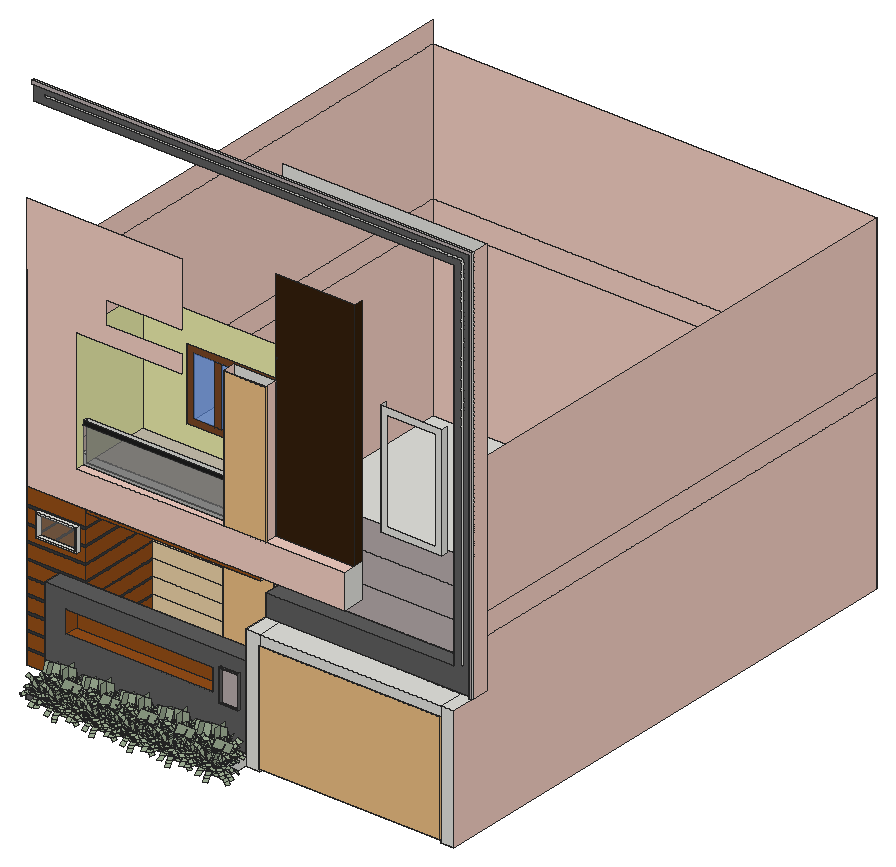
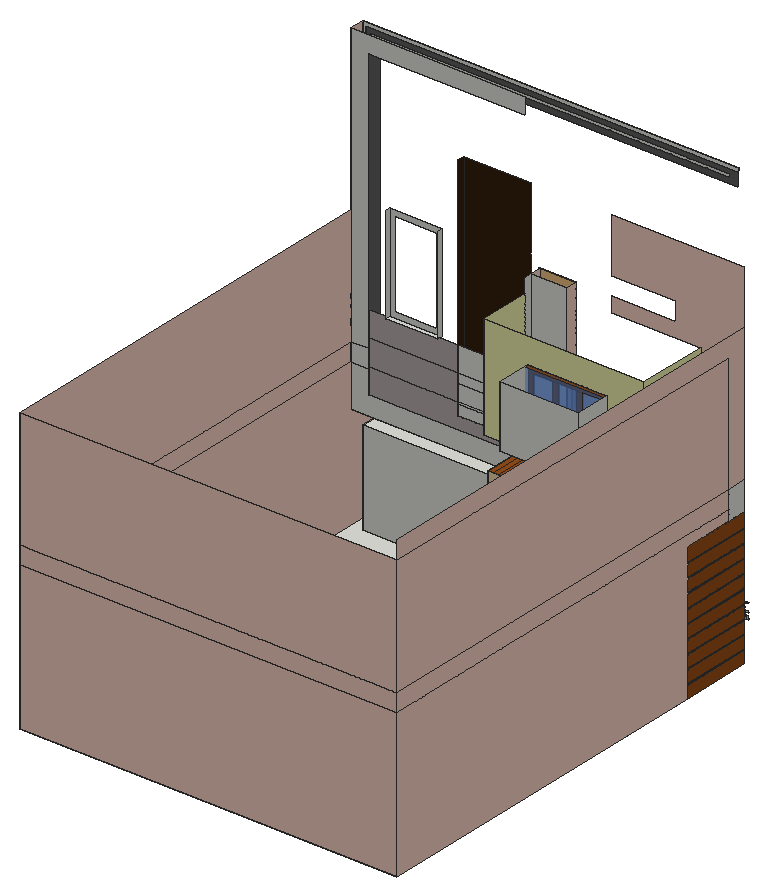
# SketchUp Ruby script. Lengths in inches.
U = 1.inch
M = Sketchup.active_model
def pt(a) = Geom::Point3d.new(a.map { |v| v * U })
def face(e, loops, mat)
  f = e.add_face(loops[0].map { |a| pt(a) })
  loops[1..].each { |l| e.add_face(l.map { |a| pt(a) }).erase! }
  f.material = f.back_material = mat if mat
  f
end
# faces: each face lists its corners as indices into pts; further lists are holes
def faces(e, pts, list, mat = nil) = list.each { |f| face(e, (f[0].is_a?(Array) ? f : [f]).map { |l| l.map { |i| pts[i] } }, mat) }
# xy, xz, yz: faces in a plane at the given z, y or x. An outline is a flat list of corners, or four numbers for a rectangle; further outlines are holes
def ring(l) = l.size == 4 ? [[l[0], l[1]], [l[2], l[1]], [l[2], l[3]], [l[0], l[3]]] : l.each_slice(2).to_a
def flat(e, list, mat, &to3) = list.each { |f| face(e, (f[0].is_a?(Array) ? f : [f]).map { |l| ring(l).map { |u, v| to3.(u, v) } }, mat) }
def xy(e, z, list, mat = nil) = flat(e, list, mat) { |x, y| [x, y, z] }
def xz(e, y, list, mat = nil) = flat(e, list, mat) { |x, z| [x, y, z] }
def yz(e, x, list, mat = nil) = flat(e, list, mat) { |y, z| [x, y, z] }
def lines(e, pts, list) = list.each { |a, b| e.add_line(pt(pts[a]), pt(pts[b])) }
# prism: a flat outline (further loops are holes) pulled along v
def prism(e, loops, v, mat = nil)
  f = face(e, loops, mat); d = Geom::Vector3d.new(v.map { |x| x * U })
  f.pushpull(f.normal.samedirection?(d) ? d.length : -d.length)
end
def box(e, o, s, mat = nil) = prism(e, [[o, [o[0] + s[0], o[1], o[2]], [o[0] + s[0], o[1] + s[1], o[2]], [o[0], o[1] + s[1], o[2]]]], [0, 0, s[2]], mat)
def at(x, y, z, deg = 0) = Geom::Transformation.translation(pt([x, y, z])) * Geom::Transformation.rotation(ORIGIN, Z_AXIS, deg.degrees)
def axes(o, x, y, z) = Geom::Transformation.new([*x, 0, *y, 0, *z, 0, *pt(o).to_a, 1])
def part(name) = M.definitions.add(name)
# library, detail: a bought-in or finely detailed component or shape, given as its bounding box
def library(name, o, s) = part(name).tap { |d| box(d.entities, o, s) }
def detail(e, o, s) = box(e.add_group.entities, o, s)
def put(e, d, t, mat = nil) = e.add_instance(d, t).tap { |i| i.material = mat if mat }
def group(e, t, mat = nil) = e.add_group.tap { |g| g.transformation = t; g.material = mat if mat }.entities
root = M.entities
M.materials.add("Generic").color = [94, 94, 94]
M.materials.add("Generic\#1").color = [182, 171, 171]
M.materials.add("Generic\#2").color = [218, 168, 133]
M.materials.add("Generic\#3").color = [149, 78, 23]
M.materials.add("Generic\#5").color = [242, 205, 193]
M.materials.add("Generic\#6").color = [236, 211, 167]
M.materials.add("Generic\#7").color = [235, 237, 171]
M.materials.add("[Color M07]").color = [58, 58, 58]
M.materials.add("[Color M08]").color = [30, 30, 30]
M.materials.add("[Field Square Tile]").color = [217, 201, 169]
M.materials.add("[Tile Canvas]").color = [199, 192, 173]
M.materials.add("[Translucent Glass Blue]").color = [100, 149, 237]
M.materials["[Translucent Glass Blue]"].alpha = 0.5
M.materials.add("[Translucent Glass Gray]").color = [128, 128, 128]
M.materials["[Translucent Glass Gray]"].alpha = 0.5
M.materials.add("[Wood Floor Dark]").color = [53, 32, 13]
M.materials.add("[Wood Veneer 01]").color = [120, 70, 37]
M.materials.add("hymenocallis littoralis").color = [156, 172, 146]
c1 = part("Group\#856")
xy(c1.entities,7.38,[[0,0,5.5,15.91]],"hymenocallis littoralis")
p = [[5.5,28.78,0],[5.5,26.79,3.44],[0,26.79,3.44],[0,28.78,0],[0,23.75,6],[5.5,23.75,6],
  [0,15.91,7.38],[5.5,15.91,7.38]]
faces(c1.entities,p,[[0,1,2,3],[4,2,1,5],[6,4,5,7]],"hymenocallis littoralis")
c2 = part("Group\#854")
xy(c2.entities,7.38,[[0,0,5.5,15.91],[0,15.91,5.5,23.87]],"hymenocallis littoralis")
p = [[5.5,31.07,4.3],[5.5,27.74,6.47],[0,27.74,6.47],[0,31.07,4.3],[0,23.87,7.38],[5.5,23.87,7.38]]
faces(c2.entities,p,[[0,1,2,3],[4,2,1,5]],"hymenocallis littoralis")
c3 = part("Group\#857")
xy(c3.entities,7.38,[[0,0,5.6,15.91]],"hymenocallis littoralis")
p = [[5.6,28.78,0],[5.6,26.79,3.44],[0,26.79,3.44],[0,28.78,0],[0,23.75,6],[5.6,23.75,6],
  [0,15.91,7.38],[5.6,15.91,7.38]]
faces(c3.entities,p,[[0,1,2,3],[4,2,1,5],[6,4,5,7]],"hymenocallis littoralis")
c4 = part("Group\#855")
put(c4.entities,c2,axes([6.09,8.57,-0.52],[0.446,0.85617,0.26089],[-0.18444,-0.19731,0.96283],[0.87582,-0.47754,0.0699]))
put(c4.entities,c2,axes([6.29,7.28,-1.71],[0.37058,0.92707,-0.05667],[-0.32382,0.19004,0.99128],[0.87712,-0.32925,0.34964]))
put(c4.entities,c2,axes([11.04,16.14,-0.7],[1,0,0],[0,0.16628,1.02662],[0,-1.18456,0.19186]))
c5 = part("Group\#860")
put(c5.entities,c1,axes([24.57,32.05,-1.76],[0.9552,-0.22102,-0.19681],[0.4036,0.95545,0.88585],[-0.00568,-0.67859,0.7345]))
put(c5.entities,c1,axes([23.95,29.24,-2.4],[0,1,0],[-0.76041,0,0.64945],[0.64945,0,0.76041]))
put(c5.entities,c1,axes([24.22,24.72,-0.48],[-0.70711,0.70711,0],[-0.32757,-0.32757,0.80237],[0.61237,0.61237,0.5]))
put(c5.entities,c2,axes([20.66,37.22,-0.63],[1.12361,0.03262,0.39091],[-0.43499,0.29739,0.78777],[0.09852,-1.27434,0.37535]))
put(c5.entities,c1,axes([28.75,24.45,-2.4],[-1,0,0],[0,-0.76041,0.64945],[0,0.64945,0.76041]))
put(c5.entities,c3,axes([30.4,30.98,-3.7],[0.65676,-0.72002,0.22414],[0.55667,0.66341,0.5],[-0.50871,-0.20361,0.83652]))
put(c5.entities,c3,axes([32.41,29.61,-3.7],[0.04029,-0.97372,0.22414],[0.85287,0.15038,0.5],[-0.52057,0.17102,0.83652]))
put(c5.entities,c1,axes([31.89,25.85,-1.76],[-0.92056,0.33739,-0.19681],[-0.5186,-0.89824,0.88585],[0.08952,0.67268,0.7345]))
put(c5.entities,c1,axes([25.55,34.78,-0.48],[0.86603,0.5,0],[-0.25,0.43301,0.86603],[0.43301,-0.75,0.5]))
put(c5.entities,c3,axes([20.4,16.9375,-8.07],[-0.70711,0.70711,0],[-0.35754,-0.35754,0.65422],[1.3987,1.3987,1.52882]))
put(c5.entities,c1,axes([32.86,34.14,-0.48],[0.76604,-0.64279,0],[0.32139,0.38302,0.86603],[-0.55667,-0.66341,0.5]))
put(c5.entities,c1,axes([27.15,34.7,-0.1],[0.82472,-0.17528,-0.53769],[0.53769,0.53769,0.64945],[0.17528,-0.82472,0.53769]))
put(c5.entities,c1,axes([33.58,28.77,-2.4],[0,-1,0],[0.76041,0,0.64945],[-0.64945,0,0.76041]))
put(c5.entities,c1,axes([26.43,23.87,-2.81],[-0.75126,0.04415,0.65853],[0.53769,-0.53769,0.64945],[0.38276,0.84199,0.3802]))
put(c5.entities,c1,axes([28.78,23.98,-2.4],[-1,0,0],[0,-0.76041,0.64945],[0,0.64945,0.76041]))
put(c5.entities,c1,axes([25.39,25.38,-2.4],[-0.70711,0.70711,0],[-0.53769,-0.53769,0.64945],[0.45923,0.45923,0.76041]))
put(c5.entities,c1,axes([27.32,21.63,-0.1],[-0.45923,0.70711,-0.53769],[-0.76041,0,0.64945],[0.45923,0.70711,0.53769]))
put(c5.entities,c1,axes([25.17,27.625,-1.76],[0.56416,0.80187,-0.19681],[-0.66673,0.66673,0.80532],[0.62659,-0.26057,0.7345]))
put(c5.entities,c3,axes([27.59,27.04,-3.96],[-0.8993,-0.06127,0.43301],[0.2962,-0.8138,0.5],[0.32175,0.57791,0.75]))
put(c5.entities,c3,axes([26.98,24.5,-3.18],[-0.5,0.86603,0],[-0.75,-0.43301,0.5],[0.43301,0.25,0.86603]))
put(c5.entities,c3,axes([24.55,27.74,-3.7],[0.29517,0.92878,0.22414],[-0.85287,0.15038,0.5],[0.43068,-0.33875,0.83652]))
put(c5.entities,c3,axes([24.26,29.8,-3.18],[0.76604,0.64279,0],[-0.47317,0.5639,0.425],[0.32139,-0.38302,0.86603]))
put(c5.entities,c3,axes([25.98,32.46,-3.18],[1,0,0],[0,0.86603,0.5],[0,-0.5,0.86603]))
put(c5.entities,c1,axes([28.78,33.57,-2.4],[1,0,0],[0,0.76041,0.64945],[0,-0.64945,0.76041]))
put(c5.entities,c4,at(14.99,21.38,2.5))
put(c5.entities,c2,axes([34.63,26.34,-1.46],[-0.70089,-0.70877,0.07994],[0.4756,-0.38088,0.79293],[-0.53156,0.59378,0.60405]))
put(c5.entities,c2,axes([28.14,16.92,1.8125],[-1.19719,0.6912,0],[-0.09607,-0.16641,0.94244],[0.68444,1.18549,0.17613]))
put(c5.entities,c2,axes([31.5625,35.84,0.97],[0.66765,-1.1564,0.35779],[0.04445,0.30732,0.91033],[-1.20828,-0.64496,0.17012]))
put(c5.entities,c2,axes([38.94,22.51,0.89],[-0.97932,-0.67164,-0.05202],[0.27787,-0.41401,0.90999],[-0.85985,0.93577,0.32097]))
put(c5.entities,c2,axes([38.44,21.09,1.98],[-1.02864,-0.54856,0.2395],[0.33481,0.06999,0.88388],[-0.77261,1.08328,0.06417]))
put(c5.entities,c3,axes([35.02,30.51,-1.3],[-0.17365,-0.98481,0],[0.60224,-0.10619,0.79122],[-0.7792,0.13739,0.61153]))
put(c5.entities,c3,axes([29.41,22.33,-1.3],[-0.93969,0.34202,0],[-0.20915,-0.57465,0.79122],[0.27061,0.74351,0.61153]))
put(c5.entities,c2,axes([19.64,36,-1.62],[1.18194,0.09546,0.08234],[-0.14377,0.68823,0.76313],[0.21457,-1.1326,0.62386]))
put(c5.entities,c3,axes([24.25,24.14,-1.3],[-0.34202,0.93969,0],[-0.57465,-0.20915,0.79122],[0.74351,0.27061,0.61153]))
put(c5.entities,c3,axes([25.98,34.61,-1.3],[1,0,0],[0,0.61153,0.79122],[0,-0.79122,0.61153]))
put(c5.entities,c3,axes([31.16,34.41,-1.64],[0.56518,-0.80224,-0.19234],[0.73413,0.34233,0.72935],[-0.47639,-0.50772,0.71782]))
put(c5.entities,c3,axes([40.52,26.84,-5.82],[-0.42262,-0.90631,0],[0.48019,-0.22391,0.68552],[-1.43418,0.66877,1.22305]))
put(c5.entities,c1,axes([29.86,38.42,-1.01],[0.89064,-0.37013,0.26413],[-0.03924,0.63286,1.01918],[-0.45353,-0.76487,0.45748]))
put(c5.entities,c1,axes([29.34,22.4,-0.48],[-0.99619,-0.08716,0],[0.04358,-0.4981,0.86603],[-0.07548,0.86273,0.5]))
c6 = part("Group\#858")
xz(c6.entities,10.07,[[9.07,0,10.07,31.01],[0,31.01,0,45.12,20.13,45.12,20.13,31.01,10.07,31.01,10.07,32.58,9.07,32.58,9.07,31.01]],"hymenocallis littoralis")
yz(c6.entities,10.07,[[0,31.01,20.13,45.12]],"hymenocallis littoralis")
p = [[9.57,9.2,0],[10.07,10.07,0],[10.07,10.07,31.01],[10.07,10.07,32.58],[9.57,9.2,32.58]]
faces(c6.entities,p,[[0,1,2,3,4]],"hymenocallis littoralis")
c7 = part("cây lá nắng")
put(c7.entities,c5,axes([49.26,-2.75,0],[0.63109,0.63109,0],[-0.63109,0.63109,0],[0,0,0.935]))
g1 = group(c7.entities,at(26.6,-8.68,0))
put(g1,c1,axes([-4.72,35.73,-1.65],[0.74231,0.46334,-0.18402],[-0.34827,0.85768,0.82827],[0.42467,-0.43184,0.68675]))
put(g1,c1,axes([-3.34,33.57,-2.24],[-0.63109,0.63109,0],[-0.47989,-0.47989,0.60723],[0.40986,0.40986,0.71098]))
put(g1,c1,axes([-0.3125,30.89,-0.45],[-0.8925,0,0],[0,-0.41345,0.75022],[0,0.77293,0.4675]))
put(g1,c2,axes([-10.79,39.66,-0.59],[0.68852,0.72969,0.3655],[-0.4622,-0.08684,0.73657],[0.86641,-0.74205,0.35095]))
put(g1,c1,axes([2.71,33.57,-2.24],[-0.63109,-0.63109,0],[0.47989,-0.47989,0.60723],[-0.40986,0.40986,0.71098]))
put(g1,c3,axes([-0.37,38.74,-3.46],[0.86887,-0.03992,0.20957],[-0.06737,0.76999,0.4675],[-0.19255,-0.44954,0.78214]))
put(g1,c3,axes([1.76,39.14,-3.46],[0.63993,-0.58908,0.20957],[0.44333,0.63315,0.4675],[-0.43646,-0.2206,0.78214]))
put(g1,c1,axes([3.81,36.4375,-1.65],[-0.79389,-0.36803,-0.18402],[0.23959,-0.89415,0.82827],[-0.36803,0.48102,0.68675]))
put(g1,c1,axes([-5.83,38.07,-0.45],[0.231,0.86209,0],[-0.43104,0.1155,0.80973],[0.74659,-0.20005,0.4675]))
put(g1,c3,axes([2.18,23.5625,-7.55],[-0.8925,0,0],[0,-0.45128,0.6117],[0,1.76542,1.42944]))
put(g1,c1,axes([-0.8125,42.28,-0.45],[0.8891,0.07779,0],[-0.03889,0.44455,0.80973],[0.06737,-0.76999,0.4675]))
put(g1,c1,axes([-4.76,39.03,-0.09],[0.63109,0.40986,-0.50274],[0,0.67866,0.60723],[0.63109,-0.40986,0.50274]))
put(g1,c1,axes([3.03,39.35,-2.24],[0.63109,-0.63109,0],[0.47989,0.47989,0.60723],[-0.40986,-0.40986,0.71098]))
put(g1,c1,axes([1.61,31.74,-2.625],[-0.50198,-0.44625,0.61573],[0.67866,0,0.60723],[-0.28982,0.77293,0.35549]))
put(g1,c1,axes([3.03,33.3,-2.24],[-0.63109,-0.63109,0],[0.47989,-0.47989,0.60723],[-0.40986,0.40986,0.71098]))
put(g1,c1,axes([0.01,32.04,-2.24],[-0.8925,0,0],[0,-0.67866,0.60723],[0,0.57963,0.71098]))
put(g1,c1,axes([3.59,30.89,-0.09],[-0.73607,0.15643,-0.50274],[-0.47989,-0.47989,0.60723],[-0.15643,0.73607,0.50274]))
put(g1,c1,axes([-1.55,33.32,-1.65],[-0.15002,0.86209,-0.18402],[-0.84154,0,0.75297],[0.55988,0.231,0.68675]))
put(g1,c3,axes([0.35,34.48,-3.71],[-0.52887,-0.60621,0.40487],[0.70051,-0.32665,0.4675],[-0.16166,0.56777,0.70125]))
put(g1,c3,axes([2.61,39.13,-1.74],[-0.86209,0.231,0],[-0.23031,-0.85954,0.15531],[0.03162,0.11799,0.91645]))
put(g1,c3,axes([-2.02,33,-3.46],[-0.39986,0.77243,0.20957],[-0.63315,-0.44333,0.4675],[0.48558,0.05802,0.78214]))
put(g1,c3,axes([-3.49,34.12,-2.97],[0.07779,0.8891,0],[-0.65449,0.05726,0.39737],[0.44455,-0.03889,0.80973]))
put(g1,c3,axes([-4.09,36.88,-2.97],[0.63109,0.63109,0],[-0.54654,0.54654,0.4675],[0.31555,-0.31555,0.80973]))
put(g1,c1,axes([-3.02,39.35,-2.24],[0.63109,0.63109,0],[-0.47989,0.47989,0.60723],[0.40986,-0.40986,0.71098]))
put(g1,c4,axes([-4.03,22.95,2.33],[0.63109,0.63109,0],[-0.63109,0.63109,0],[0,0,0.935]))
put(g1,c2,axes([5.24,38.48,-1.37],[0.00497,-0.88963,0.07474],[0.54052,0.05978,0.74139],[-0.71019,0.03927,0.56479]))
put(g1,c2,axes([7.08,28.4375,1.7],[-1.19175,-0.31933,0],[0.04439,-0.16565,0.88118],[-0.31621,1.1801,0.16468]))
put(g1,c2,axes([-2.7,42.54,0.91],[1.15114,-0.30845,0.33454],[-0.1659,0.22199,0.85115],[-0.3555,-1.16957,0.15907]))
put(g1,c2,axes([10.37,38.78,0.83],[-0.19417,-1.04191,-0.04864],[0.43664,-0.08592,0.85084],[-1.1332,0.04791,0.30011]))
put(g1,c2,axes([10.95,37.5625,1.85],[-0.30298,-0.99536,0.22393],[0.16713,0.25547,0.82643],[-1.17124,0.19607,0.06]))
put(g1,c3,axes([2.84,41.36,-1.22],[0.51192,-0.73109,0],[0.44708,0.31305,0.73979],[-0.57846,-0.40504,0.57178]))
put(g1,c3,axes([4.47,32.65,-1.22],[-0.80888,-0.37719,0],[0.23066,-0.49465,0.73979],[-0.29844,0.64,0.57178]))
put(g1,c2,axes([-10.32,35.12,-1.51],[0.68567,0.80616,0.07699],[-0.52507,0.3436,0.71352],[0.85019,-0.57936,0.58331]))
put(g1,c3,axes([0.07,30.54,-1.22],[-0.80888,0.37719,0],[-0.23066,-0.49465,0.73979],[0.29844,0.64,0.57178]))
put(g1,c3,axes([-5.45,38.24,-1.22],[0.63109,0.63109,0],[-0.38593,0.38593,0.73979],[0.49934,-0.49934,0.57178]))
put(g1,c3,axes([-2.05,41.38,-1.53],[0.86296,-0.14961,-0.17984],[0.24726,0.67935,0.68194],[0.01977,-0.62107,0.67116]))
put(g1,c3,axes([8.63,42.51,-5.4375],[0.30525,-0.83868,0],[0.44435,0.16173,0.64096],[-1.32716,-0.48305,1.14356]))
put(g1,c1,axes([-5.4,43.09,-0.94],[0.79566,0.32849,0.24696],[-0.42416,0.37462,0.95293],[0.19648,-0.76892,0.42774]))
put(g1,c1,axes([4.38,32.65,-0.45],[-0.57369,-0.68369,0],[0.34185,-0.28684,0.80973],[-0.5921,0.49683,0.4675]))
put(g1,c3,axes([-2,33.84,-0.15],[-0.24601,0.85793,0],[-0.85539,-0.24528,0.15531],[0.11742,0.03367,0.91645]))
put(g1,c3,axes([0.17,30.83,-4.47],[-0.24601,0.85793,0],[-0.85539,-0.24528,0.15531],[0.11742,0.03367,0.91645]))
put(g1,c3,axes([-1.97,32.18,-4.47],[0.58524,0.67383,0],[-0.67184,0.58351,0.15531],[0.09222,-0.0801,0.91645]))
put(g1,c3,axes([-2,34.71,-4.47],[0.88392,-0.12346,0],[0.12309,0.88131,0.15531],[-0.0169,-0.12098,0.91645]))
put(g1,c3,axes([0.11,36.12,-4.47],[0.37822,-0.8084,0],[0.80601,0.37711,0.15531],[-0.11064,-0.05177,0.91645]))
put(c7.entities,c6,axes([29.71,14.29,6.94],[0.425,0.73612,0],[-0.6771,0.39092,-0.33349],[-0.26859,0.15507,0.72712]))
put(c7.entities,c6,axes([42.0625,26.12,6.94],[0.85,0,0],[0,0.78185,-0.33349],[0,0.33349,0.78185]))
put(c7.entities,c5,axes([7.3125,23.0625,0],[0.8925,0,0],[0,0.8925,0],[0,0,0.935]))
put(c7.entities,c6,axes([24.4375,40.23,2.05],[0.85,0,0],[0,0.85,0],[0,0,0.85]))
c8 = part("Planting+101")
put(c8.entities,c7,axes([21.34,32.96,-4.59],[0,-0.71,0],[-0.71,0,0],[0,0,0.71]))
c9 = library("Group\#1",[0,0,0],[156.63,5.0625,95.0625])
c10 = library("Group\#3",[0,0,0],[44.14,4.875,81.26])
c11 = library("Leaf+Pattern+Wood+Wall+Panel (1)",[0,0,0],[40.87,0.59,87.01])
xy(root,-32,[[51.0625,60.73,202.68,131.85]],"[Field Square Tile]")
xy(root,-28.4375,[[29,23.6,202.68,60.73],[202.68,44.29,202.68,131.85,0,131.85,0,499.98,382.6875,499.98,382.6875,44.29,371.1875,44.29,371.1875,79.98,214.56,79.98,214.56,44.29],[214.56,48.39,371.1875,79.98],[0,60.73,51.0625,131.85]])
xy(root,-25,[[31.63,26.23,200.05,41.66]])
xy(root,-18.3125,[[[29,23.6,202.68,44.29],[31.63,26.23,200.05,41.66]]])
xy(root,-13.57,[[112.48,131.85,156.48,172.6]])
xy(root,13.13,[[180.92,42.79,197.32,44.29]],"Generic")
xy(root,13.81,[[181.59,42.79,196.65,44.29]],"Generic")
xy(root,19.14,[[47.45,44.29,173.82,55.48]],"Generic\#3")
xy(root,38.26,[[47.45,44.29,173.82,55.48]],"Generic\#3")
xy(root,40.68,[[181.59,42.79,196.65,44.29]],"Generic")
xy(root,41.35,[[180.92,42.79,197.32,44.29]],"Generic")
xy(root,52.87,[[29,44.29,202.68,60.73]],"Generic")
xy(root,66.625,[[214.56,44.29,371.1875,79.98]])
xy(root,67.56,[[112.48,131.85,156.48,172.6]])
xy(root,74.71,[[10.59,57.29,45.96,60.73]])
xy(root,76.26,[[12.15,57.29,44.4,60.73]])
xy(root,77.5,[[202.68,44.29,214.56,65.66],[214.56,44.29,371.1875,65.66],[371.1875,44.29,382.6875,44.29,382.6875,63.6,379.5625,63.6,379.5625,65.66,371.1875,65.66],[379.5625,63.6,382.6875,65.66],[202.68,65.66,214.56,79.98],
  [214.56,65.66,371.1875,79.98],[371.1875,65.66,382.6875,79.98]])
xy(root,93.76,[[12.15,57.29,44.4,60.73]])
xy(root,95.32,[[10.59,57.29,45.96,60.73]])
xy(root,96.37,[[202.68,65.66,365.0625,79.98]],"Generic")
xy(root,107.3125,[[51.0625,60.73,56.56,131.85],[56.56,60.73,62.06,131.85],[62.06,60.73,67.68,131.85],[67.68,60.73,73.31,131.85],[73.31,60.73,78.93,131.85],
  [78.93,60.73,84.56,131.85],[84.56,60.73,90.18,131.85],[90.18,60.73,95.81,131.85],[95.81,60.73,101.43,131.85],[101.43,60.73,107.06,131.85],
  [107.06,60.73,112.68,131.85],[112.68,60.73,118.31,131.85],[118.31,60.73,123.93,131.85],[123.93,60.73,129.56,131.85],[129.56,60.73,135.18,131.85],
  [135.18,60.73,140.81,131.85],[140.81,60.73,146.43,131.85],[146.43,60.73,152.06,131.85],[152.06,60.73,157.68,131.85],[157.68,60.73,163.31,131.85],
  [163.31,60.73,168.93,131.85],[168.93,60.73,174.56,131.85],[174.56,60.73,180.18,131.85],[180.18,60.73,185.81,131.85],[185.81,60.73,191.43,131.85],
  [191.43,60.73,197.06,131.85],[197.06,60.73,202.68,131.85]],"Generic\#3")
xy(root,109.5625,[[0,60.73,51.0625,79.98],[51.0625,60.73,202.68,79.98],[202.68,60.73,274.66,79.98],[0,79.98,51.0625,131.85]])
xy(root,138.75,[[170.12,61.18,206.39,72.04],[43.84,70.85,170.12,70.85,170.12,72.04,206.39,72.04,206.39,79.98,43.84,79.98],[206.39,71.98,274.66,79.98]])
xy(root,138.75,[[43.84,60.73,274.66,60.73,274.66,71.98,206.39,71.98,206.39,61.18,170.12,61.18,170.12,66.48,43.84,66.48]],"Generic\#5")
xy(root,138.75,[[43.84,79.98,206.39,131.85]],"[Tile Canvas]")
xy(root,155.32,[[81.41,131.85,161.72,167.54]])
xy(root,170.1875,[[43.84,66.48,170.12,70.85]])
xy(root,171.8,[[294.65,74.6,347.95,79.98]])
xz(root,23.6,[[29,-28.4375,202.68,-18.3125]],"Generic")
xz(root,26.23,[[31.63,-25,200.05,-18.3125]])
xz(root,41.66,[[31.63,-25,200.05,-18.3125]])
xz(root,42.79,[[[180.92,13.13,197.32,41.35],[181.59,13.81,196.65,40.68]]],"Generic")
xz(root,44.29,[[202.68,-28.4375,214.56,77.5],[371.1875,-28.4375,382.6875,77.5],[214.56,66.625,371.1875,77.5]])
xz(root,44.29,[[[29,-18.3125,202.68,52.87],[47.45,19.14,173.82,38.26],[180.92,13.13,197.32,41.35]]],"Generic")
xz(root,44.29,[[181.59,13.81,196.65,40.68]],"Generic\#1")
xz(root,55.48,[[47.45,19.14,173.82,38.26]],"Generic\#3")
xz(root,57.29,[[[10.59,74.71,45.96,95.32],[12.15,76.26,44.4,93.76]]])
xz(root,60.73,[[51.0625,-32,202.68,-28.4375],[29,-28.4375,51.0625,-14.64],[51.0625,-28.4375,202.68,52.87],[29,-14.64,51.0625,-0.84],[29,-0.84,51.0625,12.96],
  [29,12.96,51.0625,26.76],[29,26.76,51.0625,40.5625],[29,40.5625,51.0625,52.36],[29,52.36,51.0625,52.87]])
xz(root,60.73,[[0,-28.4375,29,-16.64],[0,-14.64,29,-2.84],[0,-0.84,29,10.96],[0,12.96,29,24.76],[0,26.76,29,38.5625],
  [0,40.5625,29,52.36],[0,54.36,51.0625,66.16],[0,68.16,51.0625,68.16,51.0625,79.96,45.96,79.96,45.96,74.71,10.59,74.71,10.59,79.96,0,79.96],[0,81.96,10.59,93.76],[45.96,81.96,51.0625,93.76],
  [0,95.76,51.0625,109.5625],[51.0625,107.3125,202.68,109.5625]],"Generic\#3")
xz(root,60.73,[[0,109.5625,274.66,109.5625,274.66,138.75,43.84,138.75,43.84,243.9375,133.85,243.9375,133.85,258.75,68.34,258.75,68.34,277.5,133.91,277.5,133.91,332.8125,0,332.8125]],"Generic\#5")
xz(root,60.73,[[0,-16.64,29,-14.64],[0,-2.84,29,-0.84],[0,10.96,29,12.96],[0,24.76,29,26.76],[0,38.5625,29,40.5625],
  [0,52.36,29,52.36,29,52.87,51.0625,52.87,51.0625,54.36,0,54.36],[0,66.16,51.0625,68.16],[0,79.96,10.59,81.96],[45.96,79.96,51.0625,81.96],[0,93.76,10.59,93.76,10.59,95.32,45.96,95.32,45.96,93.76,51.0625,93.76,51.0625,95.76,0,95.76]],"[Color M07]")
xz(root,60.73,[[12.15,76.26,44.4,93.76]],"[Translucent Glass Gray]")
xz(root,61.18,[[170.12,138.75,206.39,258.75]],"Generic\#5")
xz(root,63.6,[[379.5625,77.5,382.6875,77.5,382.6875,423.375,2.375,423.375,2.375,420.375,379.5625,420.375]],"Generic\#1")
xz(root,65.66,[[379.5625,77.5,379.5625,420.375,2.375,420.375,2.375,423.375,382.6875,423.375,382.6875,77.5],[371.27,98.79,374.08,98.79,374.08,415.02,10.82,415.02,10.82,412.39,371.27,412.39]])
xz(root,65.66,[[[202.68,77.5,379.5625,77.5,379.5625,420.375,2.375,420.375,2.375,406.6875,365.0625,406.6875,365.0625,96.37,202.68,96.37],[371.27,98.79,371.27,412.39,10.82,412.39,10.82,415.02,374.08,415.02,374.08,98.79]]],"Generic")
xz(root,66.48,[[43.84,170.1875,170.12,173.625]],"[Color M08]")
xz(root,66.48,[[43.84,138.75,170.12,170.1875]],"[Translucent Glass Gray]")
xz(root,70.85,[[43.84,170.1875,170.12,173.625]])
xz(root,70.85,[[43.84,138.75,170.12,170.1875]],"[Translucent Glass Gray]")
xz(root,71.98,[[206.39,138.75,274.66,138.75,274.66,341.34,206.39,341.34,206.39,277.5,208.2,277.5,208.2,275.5,206.39,275.5]],"[Wood Floor Dark]")
xz(root,72.04,[[170.12,138.75,206.39,258.75]])
xz(root,74.6,[[[294.65,171.8,347.95,269.6],[299.95,177.11,342.64,264.3]]])
xz(root,79.98,[[214.56,-28.4375,371.1875,66.625],[202.68,77.5,202.68,96.37,365.0625,96.37,365.0625,120,382.6875,120,382.6875,77.5],[0,109.5625,274.66,120],[0,120,274.66,138.75],[365.0625,120,382.6875,138.75],
  [206.39,138.75,274.66,148.09],[365.0625,138.75,382.6875,138.75,382.6875,423.375,206.39,423.375,206.39,406.6875,365.0625,406.6875],[206.39,148.09,274.66,173.95]])
xz(root,79.98,[[202.68,96.37,365.0625,96.37,365.0625,122.23,274.66,122.23,274.66,109.5625,202.68,109.5625],[274.66,122.23,365.0625,148.09],[274.66,148.09,365.0625,148.09,365.0625,173.95,347.95,173.95,347.95,171.8,294.65,171.8,294.65,173.95,274.66,173.95]],"Generic\#1")
xz(root,131.85,[[51.0625,-32,202.68,-28.4375],[0,-28.4375,51.0625,109.5625]])
xz(root,131.85,[[156.48,-0.84,202.68,12.96],[156.48,12.96,202.68,26.76]],"Generic\#2")
xz(root,131.85,[[51.0625,-28.4375,202.68,-14.64],[51.0625,-14.64,202.68,-14.64,202.68,-0.84,156.48,-0.84,156.48,-13.57,112.48,-13.57,112.48,-0.84,51.0625,-0.84],[51.0625,-0.84,112.48,12.96],[51.0625,12.96,112.48,26.76],[51.0625,26.76,112.48,40.5625],
  [156.48,26.76,202.68,40.5625],[51.0625,40.5625,112.48,54.36],[156.48,40.5625,202.68,54.36],[51.0625,54.36,112.48,54.36,112.48,67.56,156.48,67.56,156.48,54.36,202.68,54.36,202.68,68.16,51.0625,68.16],[51.0625,68.16,202.68,81.96],
  [51.0625,81.96,202.68,95.76],[51.0625,95.76,202.68,107.3125]],"Generic\#6")
xz(root,131.85,[[[43.84,138.75,206.39,243.9375],[81.41,155.32,161.72,217.95]]],"Generic\#7")
xz(root,167.54,[[81.41,155.32,161.72,217.95]])
xz(root,172.6,[[112.48,-13.57,156.48,67.56]])
xz(root,499.98,[[0,-28.4375,382.6875,120],[0,120,382.6875,138.75],[0,138.75,382.6875,258.75]],"Generic\#5")
yz(root,0,[[60.73,109.5625,79.98,138.75]])
yz(root,0,[[60.73,-28.4375,131.85,-16.64],[60.73,-14.64,131.85,-2.84],[60.73,-0.84,131.85,10.96],[60.73,12.96,131.85,24.76],[60.73,26.76,131.85,38.5625],
  [60.73,40.5625,131.85,52.36],[60.73,54.36,131.85,66.16],[60.73,68.16,131.85,79.96],[60.73,81.96,131.85,93.76],[60.73,95.76,131.85,109.5625]],"Generic\#3")
yz(root,0,[[131.85,-28.4375,131.85,109.5625,79.98,109.5625,79.98,120,499.98,120,499.98,-28.4375],[79.98,120,499.98,138.75],[60.73,138.75,60.73,277.5,499.98,277.5,499.98,258.75,79.98,258.75,79.98,138.75],[79.98,138.75,499.98,258.75]],"Generic\#5")
yz(root,0,[[60.73,-16.64,131.85,-14.64],[60.73,-2.84,131.85,-0.84],[60.73,10.96,131.85,12.96],[60.73,24.76,131.85,26.76],[60.73,38.5625,131.85,40.5625],
  [60.73,52.36,131.85,54.36],[60.73,66.16,131.85,68.16],[60.73,79.96,131.85,81.96],[60.73,93.76,131.85,95.76]],"[Color M07]")
yz(root,10.59,[[57.29,74.71,60.73,95.32]])
yz(root,12.15,[[57.29,76.26,60.73,93.76]])
yz(root,29,[[23.6,-28.4375,23.6,-18.3125,44.29,-18.3125,44.29,52.87,60.73,52.87,60.73,-28.4375]],"Generic")
yz(root,31.63,[[26.23,-25,41.66,-18.3125]])
yz(root,43.84,[[66.48,170.1875,70.85,173.625]])
yz(root,43.84,[[60.73,138.75,66.48,138.75,66.48,173.625,70.85,173.625,70.85,138.75,131.85,138.75,131.85,243.9375,60.73,243.9375]],"Generic\#7")
yz(root,44.4,[[57.29,76.26,60.73,93.76]])
yz(root,45.96,[[57.29,74.71,60.73,95.32]])
yz(root,47.45,[[44.29,19.14,55.48,38.26]],"Generic\#3")
yz(root,51.0625,[[60.73,107.3125,131.85,109.5625]])
yz(root,51.0625,[[60.73,-28.4375,131.85,-16.64],[60.73,-14.64,131.85,-2.84],[60.73,-0.84,131.85,10.96],[60.73,12.96,131.85,24.76],[60.73,26.76,131.85,38.5625],
  [60.73,40.5625,131.85,52.36],[60.73,54.36,131.85,66.16],[60.73,68.16,131.85,79.96],[60.73,81.96,131.85,93.76],[60.73,95.76,131.85,107.3125]],"Generic\#3")
yz(root,51.0625,[[60.73,-32,131.85,-30.4375],[60.73,-30.4375,131.85,-28.4375],[60.73,-16.64,131.85,-14.64],[60.73,-2.84,131.85,-0.84],[60.73,10.96,131.85,12.96],
  [60.73,24.76,131.85,26.76],[60.73,38.5625,131.85,40.5625],[60.73,52.36,131.85,54.36],[60.73,66.16,131.85,68.16],[60.73,79.96,131.85,81.96],
  [60.73,93.76,131.85,95.76]],"[Color M07]")
yz(root,81.41,[[131.85,155.32,167.54,217.95]])
yz(root,112.48,[[131.85,-13.57,172.6,67.56]])
yz(root,156.48,[[131.85,-13.57,172.6,67.56]])
yz(root,161.72,[[131.85,155.32,167.54,217.95]])
yz(root,170.12,[[66.48,138.75,70.85,170.1875],[66.48,170.1875,70.85,173.625]])
yz(root,170.12,[[61.18,138.75,61.18,258.75,72.04,258.75,72.04,138.75,70.85,138.75,70.85,173.625,66.48,173.625,66.48,138.75]],"Generic\#5")
yz(root,173.82,[[44.29,19.14,55.48,38.26]],"Generic\#3")
yz(root,180.92,[[42.79,13.13,44.29,41.35]],"Generic")
yz(root,181.59,[[42.79,13.81,44.29,40.68]],"Generic")
yz(root,196.65,[[42.79,13.81,44.29,40.68]],"Generic")
yz(root,197.32,[[42.79,13.13,44.29,41.35]],"Generic")
yz(root,200.05,[[26.23,-25,41.66,-18.3125]])
yz(root,202.68,[[60.73,-32,131.85,-28.4375],[23.6,-28.4375,44.29,-18.3125],[44.29,-28.4375,60.73,52.87],[60.73,-28.4375,60.73,52.87,44.29,52.87,44.29,77.5,79.98,77.5,79.98,107.3125,131.85,107.3125,131.85,-28.4375],[60.73,107.3125,79.98,109.5625]])
yz(root,202.68,[[65.66,77.5,79.98,96.37]],"Generic")
yz(root,206.39,[[71.98,138.75,72.04,258.75],[72.04,138.75,79.98,258.75]])
yz(root,206.39,[[61.18,138.75,71.98,258.75]],"Generic\#5")
yz(root,206.39,[[79.98,138.75,131.85,243.9375]],"Generic\#7")
yz(root,214.56,[[44.29,-28.4375,79.98,66.625]])
yz(root,274.66,[[60.73,109.5625,79.98,138.75]])
yz(root,274.66,[[71.98,138.75,79.98,341.34]],"[Wood Floor Dark]")
yz(root,294.65,[[74.6,171.8,79.98,269.6]])
yz(root,347.95,[[74.6,171.8,79.98,269.6]])
yz(root,365.0625,[[65.66,96.37,79.98,406.6875]],"Generic")
yz(root,371.1875,[[44.29,-28.4375,79.98,66.625]])
yz(root,379.5625,[[63.6,77.5,65.66,420.375]],"Generic\#1")
yz(root,382.6875,[[63.6,77.5,65.66,423.375]])
yz(root,382.6875,[[44.29,-28.4375,499.98,-28.4375,499.98,120,79.98,120,79.98,77.5,44.29,77.5],[65.66,77.5,79.98,423.375],[79.98,120,499.98,138.75],[79.98,138.75,499.98,258.75]],"Generic\#5")
p = [[206.39,79.98,122.23],[274.66,79.98,122.23]]
lines(root,p,[[0,1]])
put(root,c8,at(48.4,20.64,-22.31,-86.131))
put(root,c8,at(81.09,20.64,-22.31,-86.131))
put(root,c8,at(113.77,20.64,-22.31,-86.131))
put(root,c8,at(146.46,20.64,-22.31,-86.131),"Generic")
put(root,c8,at(179.15,20.64,-22.31,-86.131))
put(root,c9,at(214.56,43.54,-25.92))
put(root,c10,at(112.35,131.85,-13.57))
put(root,c11,axes([170.12,60.73,138.75],[0.9,0,0],[0,0.82,0],[0,0,1.37919]),"Generic\#5")
g2 = group(root,at(81.41,131.85,155.32),"[Translucent Glass Gray]")
xy(g2,0,[[0,0,80.3125,3.5625]],"[Wood Veneer 01]")
xy(g2,62.625,[[0,0,80.3125,3.5625]],"[Wood Veneer 01]")
xz(g2,0,[[5.91,5.91,24.8,56.71],[30.71,5.91,49.6,56.71],[55.51,5.91,74.4,56.71]],"[Translucent Glass Blue]")
xz(g2,0,[[[0,0,80.3125,62.625],[5.91,5.91,74.4,56.71]],[24.8,5.91,30.71,56.71],[49.6,5.91,55.51,56.71]],"[Wood Veneer 01]")
xz(g2,3.5625,[[0,0,80.3125,62.625]],"[Translucent Glass Blue]")
yz(g2,0,[[0,0,3.5625,62.625]],"[Wood Veneer 01]")
yz(g2,80.3125,[[0,0,3.5625,62.625]],"[Wood Veneer 01]")
